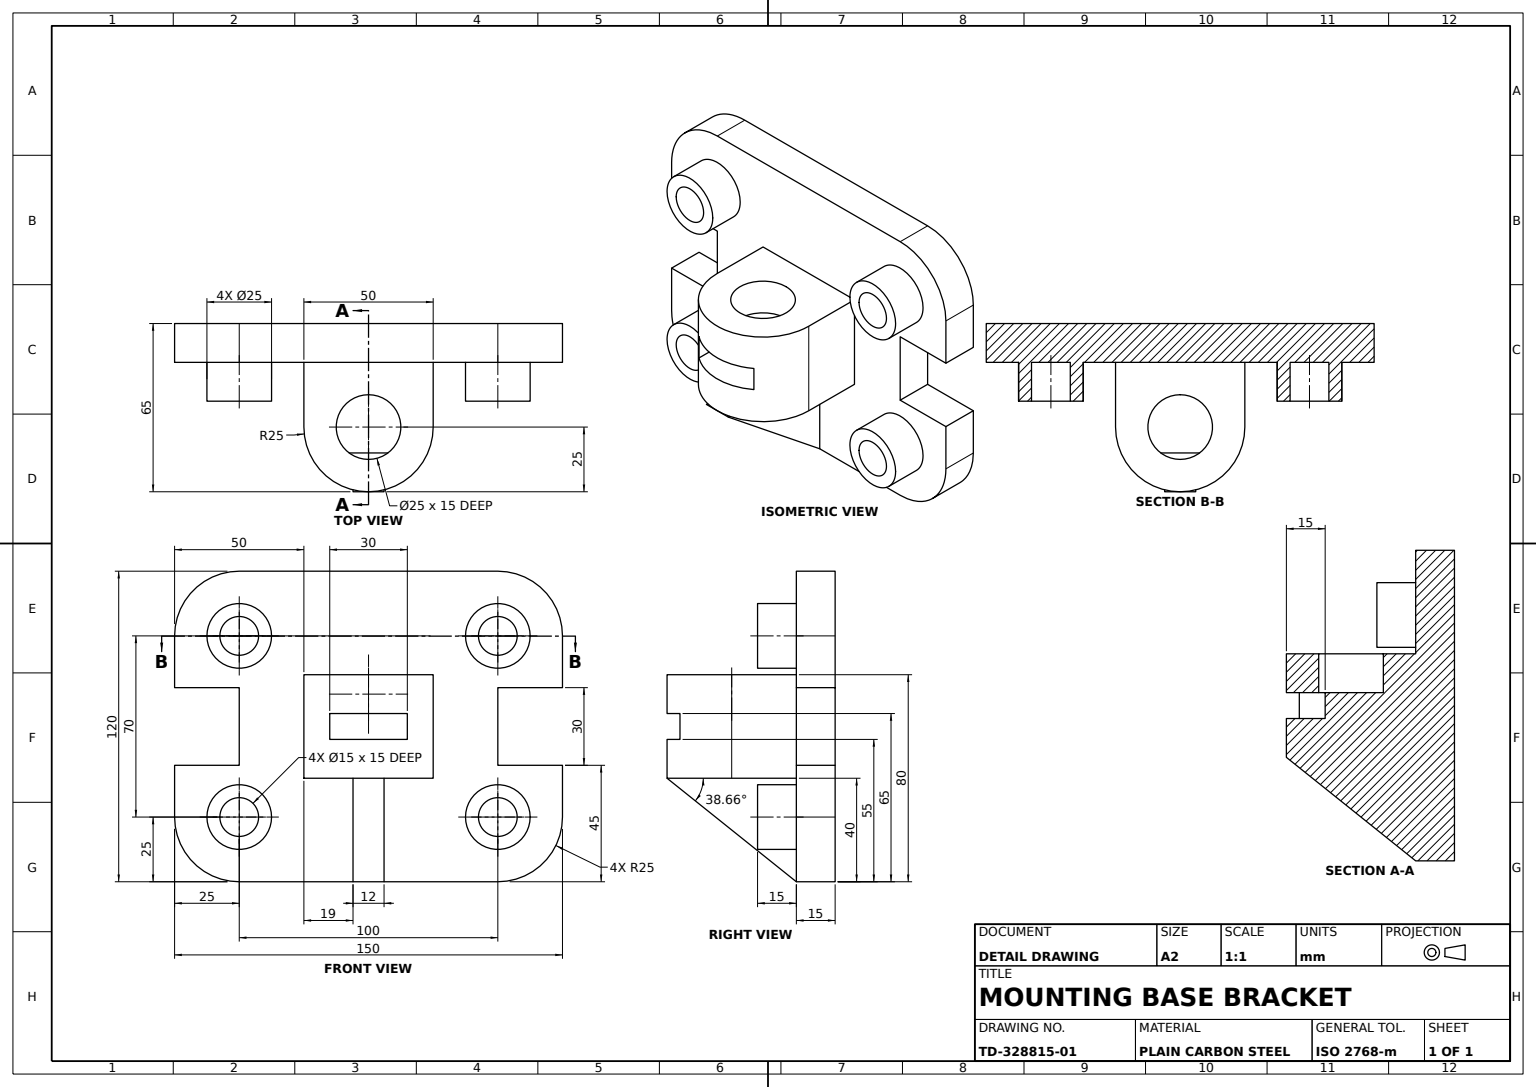
ISO-10303-21;
HEADER;
FILE_DESCRIPTION((''),'2;1');
FILE_NAME('','',(''),(''),'','','');
FILE_SCHEMA(('AUTOMOTIVE_DESIGN'));
ENDSEC;
DATA;
#1=APPLICATION_CONTEXT('');
#2=PRODUCT_CONTEXT('',#1,'mechanical');
#3=PRODUCT('','','',(#2));
#4=PRODUCT_DEFINITION_FORMATION('','',#3);
#5=PRODUCT_DEFINITION_CONTEXT('',#1,'design');
#6=PRODUCT_DEFINITION('','',#4,#5);
#7=PRODUCT_DEFINITION_SHAPE('','',#6);
#8=(LENGTH_UNIT()NAMED_UNIT(*)SI_UNIT(.MILLI.,.METRE.));
#9=(NAMED_UNIT(*)PLANE_ANGLE_UNIT()SI_UNIT($,.RADIAN.));
#10=(NAMED_UNIT(*)SI_UNIT($,.STERADIAN.)SOLID_ANGLE_UNIT());
#11=UNCERTAINTY_MEASURE_WITH_UNIT(LENGTH_MEASURE(1.E-05),#8,'distance_accuracy_value','');
#12=(GEOMETRIC_REPRESENTATION_CONTEXT(3)GLOBAL_UNCERTAINTY_ASSIGNED_CONTEXT((#11))GLOBAL_UNIT_ASSIGNED_CONTEXT((#8,#9,#10))REPRESENTATION_CONTEXT('',''));
#13=CARTESIAN_POINT('',(17.5,95.,30.));
#14=VERTEX_POINT('',#13);
#15=CARTESIAN_POINT('',(32.5,95.,30.));
#16=VERTEX_POINT('',#15);
#17=CARTESIAN_POINT('',(25.,95.,30.));
#18=DIRECTION('',(0.,0.,1.));
#19=DIRECTION('',(1.,0.,0.));
#20=AXIS2_PLACEMENT_3D('',#17,#18,#19);
#21=CIRCLE('',#20,7.5);
#22=EDGE_CURVE('',#14,#16,#21,.T.);
#23=ORIENTED_EDGE('',*,*,#22,.F.);
#24=EDGE_CURVE('',#16,#14,#21,.T.);
#25=ORIENTED_EDGE('',*,*,#24,.F.);
#26=EDGE_LOOP('',(#23,#25));
#27=FACE_BOUND('',#26,.T.);
#28=CARTESIAN_POINT('',(37.5,95.,30.));
#29=VERTEX_POINT('',#28);
#30=CARTESIAN_POINT('',(12.5,95.,30.));
#31=VERTEX_POINT('',#30);
#32=CIRCLE('',#20,12.5);
#33=EDGE_CURVE('',#29,#31,#32,.T.);
#34=ORIENTED_EDGE('',*,*,#33,.T.);
#35=EDGE_CURVE('',#31,#29,#32,.T.);
#36=ORIENTED_EDGE('',*,*,#35,.T.);
#37=EDGE_LOOP('',(#34,#36));
#38=FACE_OUTER_BOUND('',#37,.T.);
#39=PLANE('',#20);
#40=ADVANCED_FACE('',(#27,#38),#39,.T.);
#41=CARTESIAN_POINT('',(60.,65.,60.));
#42=VERTEX_POINT('',#41);
#43=CARTESIAN_POINT('',(90.,65.,60.));
#44=VERTEX_POINT('',#43);
#45=CARTESIAN_POINT('',(75.,65.,40.));
#46=DIRECTION('',(0.,1.,0.));
#47=AXIS2_PLACEMENT_3D('',#45,#46,#18);
#48=CIRCLE('',#47,25.);
#49=EDGE_CURVE('',#42,#44,#48,.T.);
#50=ORIENTED_EDGE('',*,*,#49,.F.);
#51=CARTESIAN_POINT('',(60.,65.,50.));
#52=VERTEX_POINT('',#51);
#53=VECTOR('',#18,1000.);
#54=LINE('',#51,#53);
#55=EDGE_CURVE('',#52,#42,#54,.T.);
#56=ORIENTED_EDGE('',*,*,#55,.F.);
#57=CARTESIAN_POINT('',(67.5,65.,50.));
#58=VERTEX_POINT('',#57);
#59=DIRECTION('',(-1.,0.,0.));
#60=VECTOR('',#59,1000.);
#61=LINE('',#51,#60);
#62=EDGE_CURVE('',#58,#52,#61,.T.);
#63=ORIENTED_EDGE('',*,*,#62,.F.);
#64=CARTESIAN_POINT('',(75.,65.,52.5));
#65=VERTEX_POINT('',#64);
#66=CIRCLE('',#47,12.5);
#67=EDGE_CURVE('',#58,#65,#66,.T.);
#68=ORIENTED_EDGE('',*,*,#67,.T.);
#69=CARTESIAN_POINT('',(82.5,65.,50.));
#70=VERTEX_POINT('',#69);
#71=EDGE_CURVE('',#65,#70,#66,.T.);
#72=ORIENTED_EDGE('',*,*,#71,.T.);
#73=CARTESIAN_POINT('',(90.,65.,50.));
#74=VERTEX_POINT('',#73);
#75=EDGE_CURVE('',#74,#70,#61,.T.);
#76=ORIENTED_EDGE('',*,*,#75,.F.);
#77=LINE('',#73,#53);
#78=EDGE_CURVE('',#74,#44,#77,.T.);
#79=ORIENTED_EDGE('',*,*,#78,.T.);
#80=EDGE_LOOP('',(#50,#56,#63,#68,#72,#76,#79));
#81=FACE_OUTER_BOUND('',#80,.T.);
#82=AXIS2_PLACEMENT_3D('',#51,#46,#18);
#83=PLANE('',#82);
#84=ADVANCED_FACE('',(#81),#83,.F.);
#85=CARTESIAN_POINT('',(25.,120.,15.));
#86=VERTEX_POINT('',#85);
#87=CARTESIAN_POINT('',(0.,95.,15.));
#88=VERTEX_POINT('',#87);
#89=CARTESIAN_POINT('',(25.,95.,15.));
#90=AXIS2_PLACEMENT_3D('',#89,#18,#19);
#91=CIRCLE('',#90,25.);
#92=EDGE_CURVE('',#86,#88,#91,.T.);
#93=ORIENTED_EDGE('',*,*,#92,.F.);
#94=CARTESIAN_POINT('',(25.,120.,0.));
#95=VERTEX_POINT('',#94);
#96=LINE('',#85,#53);
#97=EDGE_CURVE('',#95,#86,#96,.T.);
#98=ORIENTED_EDGE('',*,*,#97,.F.);
#99=CARTESIAN_POINT('',(0.,95.,0.));
#100=VERTEX_POINT('',#99);
#101=CARTESIAN_POINT('',(25.,95.,0.));
#102=DIRECTION('',(0.,0.,-1.));
#103=AXIS2_PLACEMENT_3D('',#101,#102,#19);
#104=CIRCLE('',#103,25.);
#105=EDGE_CURVE('',#100,#95,#104,.T.);
#106=ORIENTED_EDGE('',*,*,#105,.F.);
#107=VECTOR('',#102,1000.);
#108=LINE('',#87,#107);
#109=EDGE_CURVE('',#88,#100,#108,.T.);
#110=ORIENTED_EDGE('',*,*,#109,.F.);
#111=EDGE_LOOP('',(#93,#98,#106,#110));
#112=FACE_OUTER_BOUND('',#111,.T.);
#113=AXIS2_PLACEMENT_3D('',#89,#102,#59);
#114=CYLINDRICAL_SURFACE('',#113,25.);
#115=ADVANCED_FACE('',(#112),#114,.T.);
#116=CARTESIAN_POINT('',(81.,40.,65.));
#117=VERTEX_POINT('',#116);
#118=CARTESIAN_POINT('',(81.,0.,15.));
#119=VERTEX_POINT('',#118);
#120=DIRECTION('',(0.,-0.624695048,-0.780868809));
#121=VECTOR('',#120,1000.);
#122=LINE('',#118,#121);
#123=EDGE_CURVE('',#117,#119,#122,.T.);
#124=ORIENTED_EDGE('',*,*,#123,.T.);
#125=CARTESIAN_POINT('',(81.,40.,15.));
#126=VERTEX_POINT('',#125);
#127=VECTOR('',#46,1000.);
#128=LINE('',#125,#127);
#129=EDGE_CURVE('',#119,#126,#128,.T.);
#130=ORIENTED_EDGE('',*,*,#129,.T.);
#131=CARTESIAN_POINT('',(81.,40.,64.269322));
#132=VERTEX_POINT('',#131);
#133=LINE('',#116,#53);
#134=EDGE_CURVE('',#126,#132,#133,.T.);
#135=ORIENTED_EDGE('',*,*,#134,.T.);
#136=EDGE_CURVE('',#132,#117,#133,.T.);
#137=ORIENTED_EDGE('',*,*,#136,.T.);
#138=EDGE_LOOP('',(#124,#130,#135,#137));
#139=FACE_OUTER_BOUND('',#138,.T.);
#140=CARTESIAN_POINT('',(81.,0.,0.));
#141=AXIS2_PLACEMENT_3D('',#140,#19,#102);
#142=PLANE('',#141);
#143=ADVANCED_FACE('',(#139),#142,.T.);
#144=CARTESIAN_POINT('',(0.,25.,0.));
#145=VERTEX_POINT('',#144);
#146=CARTESIAN_POINT('',(0.,25.,15.));
#147=VERTEX_POINT('',#146);
#148=LINE('',#146,#53);
#149=EDGE_CURVE('',#145,#147,#148,.T.);
#150=ORIENTED_EDGE('',*,*,#149,.T.);
#151=CARTESIAN_POINT('',(0.,45.,15.));
#152=VERTEX_POINT('',#151);
#153=CARTESIAN_POINT('',(0.,120.,15.));
#154=DIRECTION('',(0.,-1.,0.));
#155=VECTOR('',#154,1000.);
#156=LINE('',#153,#155);
#157=EDGE_CURVE('',#152,#147,#156,.T.);
#158=ORIENTED_EDGE('',*,*,#157,.F.);
#159=CARTESIAN_POINT('',(0.,45.,0.));
#160=VERTEX_POINT('',#159);
#161=LINE('',#159,#53);
#162=EDGE_CURVE('',#160,#152,#161,.T.);
#163=ORIENTED_EDGE('',*,*,#162,.F.);
#164=CARTESIAN_POINT('',(0.,120.,0.));
#165=LINE('',#164,#155);
#166=EDGE_CURVE('',#160,#145,#165,.T.);
#167=ORIENTED_EDGE('',*,*,#166,.T.);
#168=EDGE_LOOP('',(#150,#158,#163,#167));
#169=FACE_OUTER_BOUND('',#168,.T.);
#170=AXIS2_PLACEMENT_3D('',#153,#19,#102);
#171=PLANE('',#170);
#172=ADVANCED_FACE('',(#169),#171,.F.);
#173=CARTESIAN_POINT('',(132.5,95.,30.));
#174=VERTEX_POINT('',#173);
#175=CARTESIAN_POINT('',(132.5,95.,15.));
#176=VERTEX_POINT('',#175);
#177=LINE('',#173,#107);
#178=EDGE_CURVE('',#174,#176,#177,.T.);
#179=ORIENTED_EDGE('',*,*,#178,.F.);
#180=CARTESIAN_POINT('',(117.5,95.,30.));
#181=VERTEX_POINT('',#180);
#182=CARTESIAN_POINT('',(125.,95.,30.));
#183=AXIS2_PLACEMENT_3D('',#182,#18,#19);
#184=CIRCLE('',#183,7.5);
#185=EDGE_CURVE('',#174,#181,#184,.T.);
#186=ORIENTED_EDGE('',*,*,#185,.T.);
#187=CARTESIAN_POINT('',(117.5,95.,15.));
#188=VERTEX_POINT('',#187);
#189=LINE('',#180,#107);
#190=EDGE_CURVE('',#181,#188,#189,.T.);
#191=ORIENTED_EDGE('',*,*,#190,.T.);
#192=CARTESIAN_POINT('',(125.,95.,15.));
#193=AXIS2_PLACEMENT_3D('',#192,#102,#19);
#194=CIRCLE('',#193,7.5);
#195=EDGE_CURVE('',#188,#176,#194,.T.);
#196=ORIENTED_EDGE('',*,*,#195,.T.);
#197=EDGE_LOOP('',(#179,#186,#191,#196));
#198=FACE_OUTER_BOUND('',#197,.T.);
#199=AXIS2_PLACEMENT_3D('',#182,#102,#59);
#200=CYLINDRICAL_SURFACE('',#199,7.5);
#201=ADVANCED_FACE('',(#198),#200,.F.);
#202=CARTESIAN_POINT('',(60.,55.,50.));
#203=VERTEX_POINT('',#202);
#204=LINE('',#51,#155);
#205=EDGE_CURVE('',#52,#203,#204,.T.);
#206=ORIENTED_EDGE('',*,*,#205,.F.);
#207=ORIENTED_EDGE('',*,*,#55,.T.);
#208=CARTESIAN_POINT('',(60.,55.,60.));
#209=VERTEX_POINT('',#208);
#210=CARTESIAN_POINT('',(60.,80.,60.));
#211=LINE('',#210,#127);
#212=EDGE_CURVE('',#209,#42,#211,.T.);
#213=ORIENTED_EDGE('',*,*,#212,.F.);
#214=LINE('',#202,#53);
#215=EDGE_CURVE('',#203,#209,#214,.T.);
#216=ORIENTED_EDGE('',*,*,#215,.F.);
#217=EDGE_LOOP('',(#206,#207,#213,#216));
#218=FACE_OUTER_BOUND('',#217,.T.);
#219=AXIS2_PLACEMENT_3D('',#51,#59,#18);
#220=PLANE('',#219);
#221=ADVANCED_FACE('',(#218),#220,.F.);
#222=ORIENTED_EDGE('',*,*,#109,.T.);
#223=CARTESIAN_POINT('',(0.,75.,0.));
#224=VERTEX_POINT('',#223);
#225=EDGE_CURVE('',#100,#224,#165,.T.);
#226=ORIENTED_EDGE('',*,*,#225,.T.);
#227=CARTESIAN_POINT('',(0.,75.,15.));
#228=VERTEX_POINT('',#227);
#229=LINE('',#223,#53);
#230=EDGE_CURVE('',#224,#228,#229,.T.);
#231=ORIENTED_EDGE('',*,*,#230,.T.);
#232=EDGE_CURVE('',#88,#228,#156,.T.);
#233=ORIENTED_EDGE('',*,*,#232,.F.);
#234=EDGE_LOOP('',(#222,#226,#231,#233));
#235=FACE_OUTER_BOUND('',#234,.T.);
#236=ADVANCED_FACE('',(#235),#171,.F.);
#237=CARTESIAN_POINT('',(125.,120.,15.));
#238=VERTEX_POINT('',#237);
#239=CARTESIAN_POINT('',(125.,120.,0.));
#240=VERTEX_POINT('',#239);
#241=LINE('',#237,#107);
#242=EDGE_CURVE('',#238,#240,#241,.T.);
#243=ORIENTED_EDGE('',*,*,#242,.T.);
#244=CARTESIAN_POINT('',(150.,120.,0.));
#245=LINE('',#244,#60);
#246=EDGE_CURVE('',#240,#95,#245,.T.);
#247=ORIENTED_EDGE('',*,*,#246,.T.);
#248=ORIENTED_EDGE('',*,*,#97,.T.);
#249=CARTESIAN_POINT('',(150.,120.,15.));
#250=LINE('',#249,#60);
#251=EDGE_CURVE('',#238,#86,#250,.T.);
#252=ORIENTED_EDGE('',*,*,#251,.F.);
#253=EDGE_LOOP('',(#243,#247,#248,#252));
#254=FACE_OUTER_BOUND('',#253,.T.);
#255=AXIS2_PLACEMENT_3D('',#249,#154,#102);
#256=PLANE('',#255);
#257=ADVANCED_FACE('',(#254),#256,.F.);
#258=CARTESIAN_POINT('',(25.,75.,15.));
#259=VERTEX_POINT('',#258);
#260=LINE('',#227,#60);
#261=EDGE_CURVE('',#259,#228,#260,.T.);
#262=ORIENTED_EDGE('',*,*,#261,.T.);
#263=ORIENTED_EDGE('',*,*,#230,.F.);
#264=CARTESIAN_POINT('',(25.,75.,0.));
#265=VERTEX_POINT('',#264);
#266=LINE('',#223,#60);
#267=EDGE_CURVE('',#265,#224,#266,.T.);
#268=ORIENTED_EDGE('',*,*,#267,.F.);
#269=LINE('',#264,#53);
#270=EDGE_CURVE('',#265,#259,#269,.T.);
#271=ORIENTED_EDGE('',*,*,#270,.T.);
#272=EDGE_LOOP('',(#262,#263,#268,#271));
#273=FACE_OUTER_BOUND('',#272,.T.);
#274=AXIS2_PLACEMENT_3D('',#223,#46,#18);
#275=PLANE('',#274);
#276=ADVANCED_FACE('',(#273),#275,.F.);
#277=CARTESIAN_POINT('',(100.,80.,15.));
#278=VERTEX_POINT('',#277);
#279=CARTESIAN_POINT('',(100.,40.,15.));
#280=VERTEX_POINT('',#279);
#281=LINE('',#277,#155);
#282=EDGE_CURVE('',#278,#280,#281,.T.);
#283=ORIENTED_EDGE('',*,*,#282,.F.);
#284=CARTESIAN_POINT('',(100.,80.,40.));
#285=VERTEX_POINT('',#284);
#286=LINE('',#284,#107);
#287=EDGE_CURVE('',#285,#278,#286,.T.);
#288=ORIENTED_EDGE('',*,*,#287,.F.);
#289=CARTESIAN_POINT('',(100.,40.,40.));
#290=VERTEX_POINT('',#289);
#291=LINE('',#284,#155);
#292=EDGE_CURVE('',#285,#290,#291,.T.);
#293=ORIENTED_EDGE('',*,*,#292,.T.);
#294=LINE('',#289,#107);
#295=EDGE_CURVE('',#290,#280,#294,.T.);
#296=ORIENTED_EDGE('',*,*,#295,.T.);
#297=EDGE_LOOP('',(#283,#288,#293,#296));
#298=FACE_OUTER_BOUND('',#297,.T.);
#299=AXIS2_PLACEMENT_3D('',#284,#59,#18);
#300=PLANE('',#299);
#301=ADVANCED_FACE('',(#298),#300,.F.);
#302=CARTESIAN_POINT('',(117.5,25.,15.));
#303=VERTEX_POINT('',#302);
#304=CARTESIAN_POINT('',(132.5,25.,15.));
#305=VERTEX_POINT('',#304);
#306=CARTESIAN_POINT('',(125.,25.,15.));
#307=AXIS2_PLACEMENT_3D('',#306,#102,#19);
#308=CIRCLE('',#307,7.5);
#309=EDGE_CURVE('',#303,#305,#308,.T.);
#310=ORIENTED_EDGE('',*,*,#309,.F.);
#311=EDGE_CURVE('',#305,#303,#308,.T.);
#312=ORIENTED_EDGE('',*,*,#311,.F.);
#313=EDGE_LOOP('',(#310,#312));
#314=FACE_OUTER_BOUND('',#313,.T.);
#315=CARTESIAN_POINT('',(0.,0.,15.));
#316=AXIS2_PLACEMENT_3D('',#315,#18,#19);
#317=PLANE('',#316);
#318=ADVANCED_FACE('',(#314),#317,.T.);
#319=CARTESIAN_POINT('',(125.,0.,0.));
#320=VERTEX_POINT('',#319);
#321=CARTESIAN_POINT('',(125.,0.,15.));
#322=VERTEX_POINT('',#321);
#323=LINE('',#321,#53);
#324=EDGE_CURVE('',#320,#322,#323,.T.);
#325=ORIENTED_EDGE('',*,*,#324,.F.);
#326=CARTESIAN_POINT('',(150.,25.,0.));
#327=VERTEX_POINT('',#326);
#328=CARTESIAN_POINT('',(125.,25.,0.));
#329=AXIS2_PLACEMENT_3D('',#328,#102,#19);
#330=CIRCLE('',#329,25.);
#331=EDGE_CURVE('',#327,#320,#330,.T.);
#332=ORIENTED_EDGE('',*,*,#331,.F.);
#333=CARTESIAN_POINT('',(150.,25.,15.));
#334=VERTEX_POINT('',#333);
#335=LINE('',#333,#107);
#336=EDGE_CURVE('',#334,#327,#335,.T.);
#337=ORIENTED_EDGE('',*,*,#336,.F.);
#338=AXIS2_PLACEMENT_3D('',#306,#18,#19);
#339=CIRCLE('',#338,25.);
#340=EDGE_CURVE('',#322,#334,#339,.T.);
#341=ORIENTED_EDGE('',*,*,#340,.F.);
#342=EDGE_LOOP('',(#325,#332,#337,#341));
#343=FACE_OUTER_BOUND('',#342,.T.);
#344=AXIS2_PLACEMENT_3D('',#306,#102,#59);
#345=CYLINDRICAL_SURFACE('',#344,25.);
#346=ADVANCED_FACE('',(#343),#345,.T.);
#347=CARTESIAN_POINT('',(75.,40.,65.));
#348=VERTEX_POINT('',#347);
#349=CARTESIAN_POINT('',(75.,40.,40.));
#350=AXIS2_PLACEMENT_3D('',#349,#46,#18);
#351=CIRCLE('',#350,25.);
#352=EDGE_CURVE('',#348,#132,#351,.T.);
#353=ORIENTED_EDGE('',*,*,#352,.F.);
#354=LINE('',#116,#60);
#355=EDGE_CURVE('',#117,#348,#354,.T.);
#356=ORIENTED_EDGE('',*,*,#355,.F.);
#357=ORIENTED_EDGE('',*,*,#136,.F.);
#358=EDGE_LOOP('',(#353,#356,#357));
#359=FACE_OUTER_BOUND('',#358,.T.);
#360=AXIS2_PLACEMENT_3D('',#116,#154,#102);
#361=PLANE('',#360);
#362=ADVANCED_FACE('',(#359),#361,.F.);
#363=CARTESIAN_POINT('',(90.,55.,50.));
#364=VERTEX_POINT('',#363);
#365=CARTESIAN_POINT('',(90.,55.,60.));
#366=VERTEX_POINT('',#365);
#367=LINE('',#363,#53);
#368=EDGE_CURVE('',#364,#366,#367,.T.);
#369=ORIENTED_EDGE('',*,*,#368,.F.);
#370=VECTOR('',#19,1000.);
#371=LINE('',#363,#370);
#372=EDGE_CURVE('',#203,#364,#371,.T.);
#373=ORIENTED_EDGE('',*,*,#372,.F.);
#374=ORIENTED_EDGE('',*,*,#215,.T.);
#375=CARTESIAN_POINT('',(75.,55.,40.));
#376=AXIS2_PLACEMENT_3D('',#375,#154,#102);
#377=CIRCLE('',#376,25.);
#378=EDGE_CURVE('',#366,#209,#377,.T.);
#379=ORIENTED_EDGE('',*,*,#378,.F.);
#380=EDGE_LOOP('',(#369,#373,#374,#379));
#381=FACE_OUTER_BOUND('',#380,.T.);
#382=AXIS2_PLACEMENT_3D('',#363,#154,#102);
#383=PLANE('',#382);
#384=ADVANCED_FACE('',(#381),#383,.F.);
#385=CARTESIAN_POINT('',(17.5,95.,15.));
#386=VERTEX_POINT('',#385);
#387=CARTESIAN_POINT('',(32.5,95.,15.));
#388=VERTEX_POINT('',#387);
#389=AXIS2_PLACEMENT_3D('',#89,#102,#19);
#390=CIRCLE('',#389,7.5);
#391=EDGE_CURVE('',#386,#388,#390,.T.);
#392=ORIENTED_EDGE('',*,*,#391,.T.);
#393=LINE('',#15,#107);
#394=EDGE_CURVE('',#16,#388,#393,.T.);
#395=ORIENTED_EDGE('',*,*,#394,.F.);
#396=ORIENTED_EDGE('',*,*,#24,.T.);
#397=LINE('',#13,#107);
#398=EDGE_CURVE('',#14,#386,#397,.T.);
#399=ORIENTED_EDGE('',*,*,#398,.T.);
#400=EDGE_LOOP('',(#392,#395,#396,#399));
#401=FACE_OUTER_BOUND('',#400,.T.);
#402=AXIS2_PLACEMENT_3D('',#17,#102,#59);
#403=CYLINDRICAL_SURFACE('',#402,7.5);
#404=ADVANCED_FACE('',(#401),#403,.F.);
#405=ORIENTED_EDGE('',*,*,#295,.F.);
#406=EDGE_CURVE('',#132,#290,#351,.T.);
#407=ORIENTED_EDGE('',*,*,#406,.F.);
#408=ORIENTED_EDGE('',*,*,#134,.F.);
#409=CARTESIAN_POINT('',(50.,40.,15.));
#410=LINE('',#409,#60);
#411=EDGE_CURVE('',#280,#126,#410,.T.);
#412=ORIENTED_EDGE('',*,*,#411,.F.);
#413=EDGE_LOOP('',(#405,#407,#408,#412));
#414=FACE_OUTER_BOUND('',#413,.T.);
#415=PLANE('',#350);
#416=ADVANCED_FACE('',(#414),#415,.F.);
#417=CARTESIAN_POINT('',(75.,80.,52.5));
#418=VERTEX_POINT('',#417);
#419=LINE('',#64,#127);
#420=EDGE_CURVE('',#65,#418,#419,.T.);
#421=ORIENTED_EDGE('',*,*,#420,.T.);
#422=CARTESIAN_POINT('',(75.,80.,27.5));
#423=VERTEX_POINT('',#422);
#424=CARTESIAN_POINT('',(75.,80.,40.));
#425=AXIS2_PLACEMENT_3D('',#424,#46,#18);
#426=CIRCLE('',#425,12.5);
#427=EDGE_CURVE('',#418,#423,#426,.T.);
#428=ORIENTED_EDGE('',*,*,#427,.T.);
#429=CARTESIAN_POINT('',(75.,65.,27.5));
#430=VERTEX_POINT('',#429);
#431=LINE('',#429,#127);
#432=EDGE_CURVE('',#430,#423,#431,.T.);
#433=ORIENTED_EDGE('',*,*,#432,.F.);
#434=EDGE_CURVE('',#70,#430,#66,.T.);
#435=ORIENTED_EDGE('',*,*,#434,.F.);
#436=ORIENTED_EDGE('',*,*,#71,.F.);
#437=EDGE_LOOP('',(#421,#428,#433,#435,#436));
#438=FACE_OUTER_BOUND('',#437,.T.);
#439=CYLINDRICAL_SURFACE('',#47,12.5);
#440=ADVANCED_FACE('',(#438),#439,.F.);
#441=CARTESIAN_POINT('',(125.,45.,0.));
#442=VERTEX_POINT('',#441);
#443=CARTESIAN_POINT('',(150.,45.,0.));
#444=VERTEX_POINT('',#443);
#445=LINE('',#441,#370);
#446=EDGE_CURVE('',#442,#444,#445,.T.);
#447=ORIENTED_EDGE('',*,*,#446,.F.);
#448=CARTESIAN_POINT('',(125.,45.,15.));
#449=VERTEX_POINT('',#448);
#450=LINE('',#441,#53);
#451=EDGE_CURVE('',#442,#449,#450,.T.);
#452=ORIENTED_EDGE('',*,*,#451,.T.);
#453=CARTESIAN_POINT('',(150.,45.,15.));
#454=VERTEX_POINT('',#453);
#455=LINE('',#448,#370);
#456=EDGE_CURVE('',#449,#454,#455,.T.);
#457=ORIENTED_EDGE('',*,*,#456,.T.);
#458=LINE('',#443,#53);
#459=EDGE_CURVE('',#444,#454,#458,.T.);
#460=ORIENTED_EDGE('',*,*,#459,.F.);
#461=EDGE_LOOP('',(#447,#452,#457,#460));
#462=FACE_OUTER_BOUND('',#461,.T.);
#463=AXIS2_PLACEMENT_3D('',#441,#154,#102);
#464=PLANE('',#463);
#465=ADVANCED_FACE('',(#462),#464,.F.);
#466=CARTESIAN_POINT('',(132.5,25.,30.));
#467=VERTEX_POINT('',#466);
#468=CARTESIAN_POINT('',(117.5,25.,30.));
#469=VERTEX_POINT('',#468);
#470=CARTESIAN_POINT('',(125.,25.,30.));
#471=AXIS2_PLACEMENT_3D('',#470,#18,#19);
#472=CIRCLE('',#471,7.5);
#473=EDGE_CURVE('',#467,#469,#472,.T.);
#474=ORIENTED_EDGE('',*,*,#473,.T.);
#475=LINE('',#468,#107);
#476=EDGE_CURVE('',#469,#303,#475,.T.);
#477=ORIENTED_EDGE('',*,*,#476,.T.);
#478=ORIENTED_EDGE('',*,*,#309,.T.);
#479=LINE('',#466,#107);
#480=EDGE_CURVE('',#467,#305,#479,.T.);
#481=ORIENTED_EDGE('',*,*,#480,.F.);
#482=EDGE_LOOP('',(#474,#477,#478,#481));
#483=FACE_OUTER_BOUND('',#482,.T.);
#484=AXIS2_PLACEMENT_3D('',#470,#102,#59);
#485=CYLINDRICAL_SURFACE('',#484,7.5);
#486=ADVANCED_FACE('',(#483),#485,.F.);
#487=ORIENTED_EDGE('',*,*,#67,.F.);
#488=EDGE_CURVE('',#430,#58,#66,.T.);
#489=ORIENTED_EDGE('',*,*,#488,.F.);
#490=ORIENTED_EDGE('',*,*,#432,.T.);
#491=EDGE_CURVE('',#423,#418,#426,.T.);
#492=ORIENTED_EDGE('',*,*,#491,.T.);
#493=ORIENTED_EDGE('',*,*,#420,.F.);
#494=EDGE_LOOP('',(#487,#489,#490,#492,#493));
#495=FACE_OUTER_BOUND('',#494,.T.);
#496=ADVANCED_FACE('',(#495),#439,.F.);
#497=ORIENTED_EDGE('',*,*,#242,.F.);
#498=CARTESIAN_POINT('',(150.,95.,15.));
#499=VERTEX_POINT('',#498);
#500=AXIS2_PLACEMENT_3D('',#192,#18,#19);
#501=CIRCLE('',#500,25.);
#502=EDGE_CURVE('',#499,#238,#501,.T.);
#503=ORIENTED_EDGE('',*,*,#502,.F.);
#504=CARTESIAN_POINT('',(150.,95.,0.));
#505=VERTEX_POINT('',#504);
#506=LINE('',#498,#53);
#507=EDGE_CURVE('',#505,#499,#506,.T.);
#508=ORIENTED_EDGE('',*,*,#507,.F.);
#509=CARTESIAN_POINT('',(125.,95.,0.));
#510=AXIS2_PLACEMENT_3D('',#509,#102,#19);
#511=CIRCLE('',#510,25.);
#512=EDGE_CURVE('',#240,#505,#511,.T.);
#513=ORIENTED_EDGE('',*,*,#512,.F.);
#514=EDGE_LOOP('',(#497,#503,#508,#513));
#515=FACE_OUTER_BOUND('',#514,.T.);
#516=AXIS2_PLACEMENT_3D('',#192,#102,#59);
#517=CYLINDRICAL_SURFACE('',#516,25.);
#518=ADVANCED_FACE('',(#515),#517,.T.);
#519=ORIENTED_EDGE('',*,*,#123,.F.);
#520=ORIENTED_EDGE('',*,*,#355,.T.);
#521=CARTESIAN_POINT('',(69.,40.,65.));
#522=VERTEX_POINT('',#521);
#523=EDGE_CURVE('',#348,#522,#354,.T.);
#524=ORIENTED_EDGE('',*,*,#523,.T.);
#525=CARTESIAN_POINT('',(69.,0.,15.));
#526=VERTEX_POINT('',#525);
#527=LINE('',#525,#121);
#528=EDGE_CURVE('',#522,#526,#527,.T.);
#529=ORIENTED_EDGE('',*,*,#528,.T.);
#530=LINE('',#118,#60);
#531=EDGE_CURVE('',#119,#526,#530,.T.);
#532=ORIENTED_EDGE('',*,*,#531,.F.);
#533=EDGE_LOOP('',(#519,#520,#524,#529,#532));
#534=FACE_OUTER_BOUND('',#533,.T.);
#535=DIRECTION('',(0.,0.780868809,-0.624695048));
#536=DIRECTION('',(0.,0.624695048,0.780868809));
#537=AXIS2_PLACEMENT_3D('',#118,#535,#536);
#538=PLANE('',#537);
#539=ADVANCED_FACE('',(#534),#538,.F.);
#540=CARTESIAN_POINT('',(69.,40.,64.269322));
#541=VERTEX_POINT('',#540);
#542=EDGE_CURVE('',#541,#348,#351,.T.);
#543=ORIENTED_EDGE('',*,*,#542,.T.);
#544=ORIENTED_EDGE('',*,*,#352,.T.);
#545=ORIENTED_EDGE('',*,*,#406,.T.);
#546=ORIENTED_EDGE('',*,*,#292,.F.);
#547=CARTESIAN_POINT('',(50.,80.,40.));
#548=VERTEX_POINT('',#547);
#549=CIRCLE('',#425,25.);
#550=EDGE_CURVE('',#548,#285,#549,.T.);
#551=ORIENTED_EDGE('',*,*,#550,.F.);
#552=CARTESIAN_POINT('',(50.,40.,40.));
#553=VERTEX_POINT('',#552);
#554=LINE('',#547,#155);
#555=EDGE_CURVE('',#548,#553,#554,.T.);
#556=ORIENTED_EDGE('',*,*,#555,.T.);
#557=EDGE_CURVE('',#553,#541,#351,.T.);
#558=ORIENTED_EDGE('',*,*,#557,.T.);
#559=EDGE_LOOP('',(#543,#544,#545,#546,#551,#556,#558));
#560=FACE_OUTER_BOUND('',#559,.T.);
#561=ORIENTED_EDGE('',*,*,#212,.T.);
#562=ORIENTED_EDGE('',*,*,#49,.T.);
#563=CARTESIAN_POINT('',(90.,80.,60.));
#564=LINE('',#563,#155);
#565=EDGE_CURVE('',#44,#366,#564,.T.);
#566=ORIENTED_EDGE('',*,*,#565,.T.);
#567=ORIENTED_EDGE('',*,*,#378,.T.);
#568=EDGE_LOOP('',(#561,#562,#566,#567));
#569=FACE_BOUND('',#568,.T.);
#570=AXIS2_PLACEMENT_3D('',#424,#154,#102);
#571=CYLINDRICAL_SURFACE('',#570,25.);
#572=ADVANCED_FACE('',(#560,#569),#571,.T.);
#573=CARTESIAN_POINT('',(112.5,25.,15.));
#574=VERTEX_POINT('',#573);
#575=CARTESIAN_POINT('',(137.5,25.,15.));
#576=VERTEX_POINT('',#575);
#577=CIRCLE('',#338,12.5);
#578=EDGE_CURVE('',#574,#576,#577,.T.);
#579=ORIENTED_EDGE('',*,*,#578,.T.);
#580=CARTESIAN_POINT('',(137.5,25.,30.));
#581=VERTEX_POINT('',#580);
#582=LINE('',#580,#107);
#583=EDGE_CURVE('',#581,#576,#582,.T.);
#584=ORIENTED_EDGE('',*,*,#583,.F.);
#585=CARTESIAN_POINT('',(112.5,25.,30.));
#586=VERTEX_POINT('',#585);
#587=CIRCLE('',#471,12.5);
#588=EDGE_CURVE('',#586,#581,#587,.T.);
#589=ORIENTED_EDGE('',*,*,#588,.F.);
#590=LINE('',#585,#107);
#591=EDGE_CURVE('',#586,#574,#590,.T.);
#592=ORIENTED_EDGE('',*,*,#591,.T.);
#593=EDGE_LOOP('',(#579,#584,#589,#592));
#594=FACE_OUTER_BOUND('',#593,.T.);
#595=CYLINDRICAL_SURFACE('',#484,12.5);
#596=ADVANCED_FACE('',(#594),#595,.T.);
#597=ORIENTED_EDGE('',*,*,#33,.F.);
#598=CARTESIAN_POINT('',(37.5,95.,15.));
#599=VERTEX_POINT('',#598);
#600=LINE('',#28,#107);
#601=EDGE_CURVE('',#29,#599,#600,.T.);
#602=ORIENTED_EDGE('',*,*,#601,.T.);
#603=CARTESIAN_POINT('',(12.5,95.,15.));
#604=VERTEX_POINT('',#603);
#605=CIRCLE('',#90,12.5);
#606=EDGE_CURVE('',#599,#604,#605,.T.);
#607=ORIENTED_EDGE('',*,*,#606,.T.);
#608=LINE('',#30,#107);
#609=EDGE_CURVE('',#31,#604,#608,.T.);
#610=ORIENTED_EDGE('',*,*,#609,.F.);
#611=EDGE_LOOP('',(#597,#602,#607,#610));
#612=FACE_OUTER_BOUND('',#611,.T.);
#613=CYLINDRICAL_SURFACE('',#402,12.5);
#614=ADVANCED_FACE('',(#612),#613,.T.);
#615=ORIENTED_EDGE('',*,*,#609,.T.);
#616=EDGE_CURVE('',#604,#599,#605,.T.);
#617=ORIENTED_EDGE('',*,*,#616,.T.);
#618=ORIENTED_EDGE('',*,*,#601,.F.);
#619=ORIENTED_EDGE('',*,*,#35,.F.);
#620=EDGE_LOOP('',(#615,#617,#618,#619));
#621=FACE_OUTER_BOUND('',#620,.T.);
#622=ADVANCED_FACE('',(#621),#613,.T.);
#623=CARTESIAN_POINT('',(112.5,95.,30.));
#624=VERTEX_POINT('',#623);
#625=CARTESIAN_POINT('',(112.5,95.,15.));
#626=VERTEX_POINT('',#625);
#627=LINE('',#623,#107);
#628=EDGE_CURVE('',#624,#626,#627,.T.);
#629=ORIENTED_EDGE('',*,*,#628,.T.);
#630=CARTESIAN_POINT('',(137.5,95.,15.));
#631=VERTEX_POINT('',#630);
#632=CIRCLE('',#500,12.5);
#633=EDGE_CURVE('',#626,#631,#632,.T.);
#634=ORIENTED_EDGE('',*,*,#633,.T.);
#635=CARTESIAN_POINT('',(137.5,95.,30.));
#636=VERTEX_POINT('',#635);
#637=LINE('',#635,#107);
#638=EDGE_CURVE('',#636,#631,#637,.T.);
#639=ORIENTED_EDGE('',*,*,#638,.F.);
#640=CIRCLE('',#183,12.5);
#641=EDGE_CURVE('',#624,#636,#640,.T.);
#642=ORIENTED_EDGE('',*,*,#641,.F.);
#643=EDGE_LOOP('',(#629,#634,#639,#642));
#644=FACE_OUTER_BOUND('',#643,.T.);
#645=CYLINDRICAL_SURFACE('',#199,12.5);
#646=ADVANCED_FACE('',(#644),#645,.T.);
#647=CARTESIAN_POINT('',(12.5,25.,30.));
#648=VERTEX_POINT('',#647);
#649=CARTESIAN_POINT('',(37.5,25.,30.));
#650=VERTEX_POINT('',#649);
#651=CARTESIAN_POINT('',(25.,25.,30.));
#652=AXIS2_PLACEMENT_3D('',#651,#18,#19);
#653=CIRCLE('',#652,12.5);
#654=EDGE_CURVE('',#648,#650,#653,.T.);
#655=ORIENTED_EDGE('',*,*,#654,.F.);
#656=CARTESIAN_POINT('',(12.5,25.,15.));
#657=VERTEX_POINT('',#656);
#658=LINE('',#647,#107);
#659=EDGE_CURVE('',#648,#657,#658,.T.);
#660=ORIENTED_EDGE('',*,*,#659,.T.);
#661=CARTESIAN_POINT('',(37.5,25.,15.));
#662=VERTEX_POINT('',#661);
#663=CARTESIAN_POINT('',(25.,25.,15.));
#664=AXIS2_PLACEMENT_3D('',#663,#18,#19);
#665=CIRCLE('',#664,12.5);
#666=EDGE_CURVE('',#657,#662,#665,.T.);
#667=ORIENTED_EDGE('',*,*,#666,.T.);
#668=LINE('',#649,#107);
#669=EDGE_CURVE('',#650,#662,#668,.T.);
#670=ORIENTED_EDGE('',*,*,#669,.F.);
#671=EDGE_LOOP('',(#655,#660,#667,#670));
#672=FACE_OUTER_BOUND('',#671,.T.);
#673=AXIS2_PLACEMENT_3D('',#651,#102,#59);
#674=CYLINDRICAL_SURFACE('',#673,12.5);
#675=ADVANCED_FACE('',(#672),#674,.T.);
#676=CARTESIAN_POINT('',(25.,45.,0.));
#677=VERTEX_POINT('',#676);
#678=LINE('',#264,#127);
#679=EDGE_CURVE('',#677,#265,#678,.T.);
#680=ORIENTED_EDGE('',*,*,#679,.F.);
#681=CARTESIAN_POINT('',(25.,45.,15.));
#682=VERTEX_POINT('',#681);
#683=LINE('',#676,#53);
#684=EDGE_CURVE('',#677,#682,#683,.T.);
#685=ORIENTED_EDGE('',*,*,#684,.T.);
#686=LINE('',#258,#127);
#687=EDGE_CURVE('',#682,#259,#686,.T.);
#688=ORIENTED_EDGE('',*,*,#687,.T.);
#689=ORIENTED_EDGE('',*,*,#270,.F.);
#690=EDGE_LOOP('',(#680,#685,#688,#689));
#691=FACE_OUTER_BOUND('',#690,.T.);
#692=AXIS2_PLACEMENT_3D('',#264,#19,#102);
#693=PLANE('',#692);
#694=ADVANCED_FACE('',(#691),#693,.F.);
#695=EDGE_CURVE('',#176,#188,#194,.T.);
#696=ORIENTED_EDGE('',*,*,#695,.T.);
#697=ORIENTED_EDGE('',*,*,#190,.F.);
#698=EDGE_CURVE('',#181,#174,#184,.T.);
#699=ORIENTED_EDGE('',*,*,#698,.T.);
#700=ORIENTED_EDGE('',*,*,#178,.T.);
#701=EDGE_LOOP('',(#696,#697,#699,#700));
#702=FACE_OUTER_BOUND('',#701,.T.);
#703=ADVANCED_FACE('',(#702),#200,.F.);
#704=CARTESIAN_POINT('',(32.5,25.,30.));
#705=VERTEX_POINT('',#704);
#706=CARTESIAN_POINT('',(17.5,25.,30.));
#707=VERTEX_POINT('',#706);
#708=CIRCLE('',#652,7.5);
#709=EDGE_CURVE('',#705,#707,#708,.T.);
#710=ORIENTED_EDGE('',*,*,#709,.F.);
#711=EDGE_CURVE('',#707,#705,#708,.T.);
#712=ORIENTED_EDGE('',*,*,#711,.F.);
#713=EDGE_LOOP('',(#710,#712));
#714=FACE_BOUND('',#713,.T.);
#715=ORIENTED_EDGE('',*,*,#654,.T.);
#716=EDGE_CURVE('',#650,#648,#653,.T.);
#717=ORIENTED_EDGE('',*,*,#716,.T.);
#718=EDGE_LOOP('',(#715,#717));
#719=FACE_OUTER_BOUND('',#718,.T.);
#720=PLANE('',#652);
#721=ADVANCED_FACE('',(#714,#719),#720,.T.);
#722=EDGE_CURVE('',#469,#467,#472,.T.);
#723=ORIENTED_EDGE('',*,*,#722,.T.);
#724=ORIENTED_EDGE('',*,*,#480,.T.);
#725=ORIENTED_EDGE('',*,*,#311,.T.);
#726=ORIENTED_EDGE('',*,*,#476,.F.);
#727=EDGE_LOOP('',(#723,#724,#725,#726));
#728=FACE_OUTER_BOUND('',#727,.T.);
#729=ADVANCED_FACE('',(#728),#485,.F.);
#730=ORIENTED_EDGE('',*,*,#666,.F.);
#731=EDGE_CURVE('',#662,#657,#665,.T.);
#732=ORIENTED_EDGE('',*,*,#731,.F.);
#733=EDGE_LOOP('',(#730,#732));
#734=FACE_BOUND('',#733,.T.);
#735=EDGE_CURVE('',#631,#626,#632,.T.);
#736=ORIENTED_EDGE('',*,*,#735,.F.);
#737=ORIENTED_EDGE('',*,*,#633,.F.);
#738=EDGE_LOOP('',(#736,#737));
#739=FACE_BOUND('',#738,.T.);
#740=EDGE_CURVE('',#576,#574,#577,.T.);
#741=ORIENTED_EDGE('',*,*,#740,.F.);
#742=ORIENTED_EDGE('',*,*,#578,.F.);
#743=EDGE_LOOP('',(#741,#742));
#744=FACE_BOUND('',#743,.T.);
#745=ORIENTED_EDGE('',*,*,#606,.F.);
#746=ORIENTED_EDGE('',*,*,#616,.F.);
#747=EDGE_LOOP('',(#745,#746));
#748=FACE_BOUND('',#747,.T.);
#749=ORIENTED_EDGE('',*,*,#340,.T.);
#750=CARTESIAN_POINT('',(150.,0.,15.));
#751=LINE('',#750,#127);
#752=EDGE_CURVE('',#334,#454,#751,.T.);
#753=ORIENTED_EDGE('',*,*,#752,.T.);
#754=ORIENTED_EDGE('',*,*,#456,.F.);
#755=CARTESIAN_POINT('',(125.,75.,15.));
#756=VERTEX_POINT('',#755);
#757=LINE('',#755,#155);
#758=EDGE_CURVE('',#756,#449,#757,.T.);
#759=ORIENTED_EDGE('',*,*,#758,.F.);
#760=CARTESIAN_POINT('',(150.,75.,15.));
#761=VERTEX_POINT('',#760);
#762=LINE('',#760,#60);
#763=EDGE_CURVE('',#761,#756,#762,.T.);
#764=ORIENTED_EDGE('',*,*,#763,.F.);
#765=EDGE_CURVE('',#761,#499,#751,.T.);
#766=ORIENTED_EDGE('',*,*,#765,.T.);
#767=ORIENTED_EDGE('',*,*,#502,.T.);
#768=ORIENTED_EDGE('',*,*,#251,.T.);
#769=ORIENTED_EDGE('',*,*,#92,.T.);
#770=ORIENTED_EDGE('',*,*,#232,.T.);
#771=ORIENTED_EDGE('',*,*,#261,.F.);
#772=ORIENTED_EDGE('',*,*,#687,.F.);
#773=LINE('',#681,#370);
#774=EDGE_CURVE('',#152,#682,#773,.T.);
#775=ORIENTED_EDGE('',*,*,#774,.F.);
#776=ORIENTED_EDGE('',*,*,#157,.T.);
#777=CARTESIAN_POINT('',(25.,0.,15.));
#778=VERTEX_POINT('',#777);
#779=CIRCLE('',#664,25.);
#780=EDGE_CURVE('',#147,#778,#779,.T.);
#781=ORIENTED_EDGE('',*,*,#780,.T.);
#782=LINE('',#315,#370);
#783=EDGE_CURVE('',#778,#526,#782,.T.);
#784=ORIENTED_EDGE('',*,*,#783,.T.);
#785=CARTESIAN_POINT('',(69.,40.,15.));
#786=VERTEX_POINT('',#785);
#787=LINE('',#785,#127);
#788=EDGE_CURVE('',#526,#786,#787,.T.);
#789=ORIENTED_EDGE('',*,*,#788,.T.);
#790=VERTEX_POINT('',#409);
#791=EDGE_CURVE('',#786,#790,#410,.T.);
#792=ORIENTED_EDGE('',*,*,#791,.T.);
#793=CARTESIAN_POINT('',(50.,80.,15.));
#794=VERTEX_POINT('',#793);
#795=LINE('',#793,#155);
#796=EDGE_CURVE('',#794,#790,#795,.T.);
#797=ORIENTED_EDGE('',*,*,#796,.F.);
#798=LINE('',#793,#60);
#799=EDGE_CURVE('',#278,#794,#798,.T.);
#800=ORIENTED_EDGE('',*,*,#799,.F.);
#801=ORIENTED_EDGE('',*,*,#282,.T.);
#802=ORIENTED_EDGE('',*,*,#411,.T.);
#803=ORIENTED_EDGE('',*,*,#129,.F.);
#804=EDGE_CURVE('',#119,#322,#782,.T.);
#805=ORIENTED_EDGE('',*,*,#804,.T.);
#806=EDGE_LOOP('',(#749,#753,#754,#759,#764,#766,#767,#768,#769,#770,#771,#772,#775,#776,#781,#784,#789,#792,#797,#800,#801,#802,#803,#805));
#807=FACE_OUTER_BOUND('',#806,.T.);
#808=ADVANCED_FACE('',(#734,#739,#744,#748,#807),#317,.T.);
#809=ORIENTED_EDGE('',*,*,#695,.F.);
#810=ORIENTED_EDGE('',*,*,#195,.F.);
#811=EDGE_LOOP('',(#809,#810));
#812=FACE_OUTER_BOUND('',#811,.T.);
#813=ADVANCED_FACE('',(#812),#317,.T.);
#814=ORIENTED_EDGE('',*,*,#398,.F.);
#815=ORIENTED_EDGE('',*,*,#22,.T.);
#816=ORIENTED_EDGE('',*,*,#394,.T.);
#817=EDGE_CURVE('',#388,#386,#390,.T.);
#818=ORIENTED_EDGE('',*,*,#817,.T.);
#819=EDGE_LOOP('',(#814,#815,#816,#818));
#820=FACE_OUTER_BOUND('',#819,.T.);
#821=ADVANCED_FACE('',(#820),#403,.F.);
#822=ORIENTED_EDGE('',*,*,#166,.F.);
#823=LINE('',#676,#370);
#824=EDGE_CURVE('',#160,#677,#823,.T.);
#825=ORIENTED_EDGE('',*,*,#824,.T.);
#826=ORIENTED_EDGE('',*,*,#679,.T.);
#827=ORIENTED_EDGE('',*,*,#267,.T.);
#828=ORIENTED_EDGE('',*,*,#225,.F.);
#829=ORIENTED_EDGE('',*,*,#105,.T.);
#830=ORIENTED_EDGE('',*,*,#246,.F.);
#831=ORIENTED_EDGE('',*,*,#512,.T.);
#832=CARTESIAN_POINT('',(150.,75.,0.));
#833=VERTEX_POINT('',#832);
#834=CARTESIAN_POINT('',(150.,0.,0.));
#835=LINE('',#834,#127);
#836=EDGE_CURVE('',#833,#505,#835,.T.);
#837=ORIENTED_EDGE('',*,*,#836,.F.);
#838=CARTESIAN_POINT('',(125.,75.,0.));
#839=VERTEX_POINT('',#838);
#840=LINE('',#832,#60);
#841=EDGE_CURVE('',#833,#839,#840,.T.);
#842=ORIENTED_EDGE('',*,*,#841,.T.);
#843=LINE('',#838,#155);
#844=EDGE_CURVE('',#839,#442,#843,.T.);
#845=ORIENTED_EDGE('',*,*,#844,.T.);
#846=ORIENTED_EDGE('',*,*,#446,.T.);
#847=EDGE_CURVE('',#327,#444,#835,.T.);
#848=ORIENTED_EDGE('',*,*,#847,.F.);
#849=ORIENTED_EDGE('',*,*,#331,.T.);
#850=CARTESIAN_POINT('',(25.,0.,0.));
#851=VERTEX_POINT('',#850);
#852=CARTESIAN_POINT('',(0.,0.,0.));
#853=LINE('',#852,#370);
#854=EDGE_CURVE('',#851,#320,#853,.T.);
#855=ORIENTED_EDGE('',*,*,#854,.F.);
#856=CARTESIAN_POINT('',(25.,25.,0.));
#857=AXIS2_PLACEMENT_3D('',#856,#102,#19);
#858=CIRCLE('',#857,25.);
#859=EDGE_CURVE('',#851,#145,#858,.T.);
#860=ORIENTED_EDGE('',*,*,#859,.T.);
#861=EDGE_LOOP('',(#822,#825,#826,#827,#828,#829,#830,#831,#837,#842,#845,#846,#848,#849,#855,#860));
#862=FACE_OUTER_BOUND('',#861,.T.);
#863=AXIS2_PLACEMENT_3D('',#852,#18,#19);
#864=PLANE('',#863);
#865=ADVANCED_FACE('',(#862),#864,.F.);
#866=EDGE_CURVE('',#636,#624,#640,.T.);
#867=ORIENTED_EDGE('',*,*,#866,.T.);
#868=ORIENTED_EDGE('',*,*,#641,.T.);
#869=EDGE_LOOP('',(#867,#868));
#870=FACE_OUTER_BOUND('',#869,.T.);
#871=ORIENTED_EDGE('',*,*,#185,.F.);
#872=ORIENTED_EDGE('',*,*,#698,.F.);
#873=EDGE_LOOP('',(#871,#872));
#874=FACE_BOUND('',#873,.T.);
#875=PLANE('',#183);
#876=ADVANCED_FACE('',(#870,#874),#875,.T.);
#877=ORIENTED_EDGE('',*,*,#488,.T.);
#878=EDGE_CURVE('',#70,#58,#61,.T.);
#879=ORIENTED_EDGE('',*,*,#878,.F.);
#880=ORIENTED_EDGE('',*,*,#434,.T.);
#881=EDGE_LOOP('',(#877,#879,#880));
#882=FACE_OUTER_BOUND('',#881,.T.);
#883=PLANE('',#47);
#884=ADVANCED_FACE('',(#882),#883,.T.);
#885=ORIENTED_EDGE('',*,*,#752,.F.);
#886=ORIENTED_EDGE('',*,*,#336,.T.);
#887=ORIENTED_EDGE('',*,*,#847,.T.);
#888=ORIENTED_EDGE('',*,*,#459,.T.);
#889=EDGE_LOOP('',(#885,#886,#887,#888));
#890=FACE_OUTER_BOUND('',#889,.T.);
#891=AXIS2_PLACEMENT_3D('',#750,#59,#18);
#892=PLANE('',#891);
#893=ADVANCED_FACE('',(#890),#892,.F.);
#894=ORIENTED_EDGE('',*,*,#324,.T.);
#895=ORIENTED_EDGE('',*,*,#804,.F.);
#896=ORIENTED_EDGE('',*,*,#531,.T.);
#897=ORIENTED_EDGE('',*,*,#783,.F.);
#898=LINE('',#777,#107);
#899=EDGE_CURVE('',#778,#851,#898,.T.);
#900=ORIENTED_EDGE('',*,*,#899,.T.);
#901=ORIENTED_EDGE('',*,*,#854,.T.);
#902=EDGE_LOOP('',(#894,#895,#896,#897,#900,#901));
#903=FACE_OUTER_BOUND('',#902,.T.);
#904=AXIS2_PLACEMENT_3D('',#315,#46,#18);
#905=PLANE('',#904);
#906=ADVANCED_FACE('',(#903),#905,.F.);
#907=ORIENTED_EDGE('',*,*,#287,.T.);
#908=ORIENTED_EDGE('',*,*,#799,.T.);
#909=LINE('',#547,#53);
#910=EDGE_CURVE('',#794,#548,#909,.T.);
#911=ORIENTED_EDGE('',*,*,#910,.T.);
#912=ORIENTED_EDGE('',*,*,#550,.T.);
#913=EDGE_LOOP('',(#907,#908,#911,#912));
#914=FACE_OUTER_BOUND('',#913,.T.);
#915=ORIENTED_EDGE('',*,*,#427,.F.);
#916=ORIENTED_EDGE('',*,*,#491,.F.);
#917=EDGE_LOOP('',(#915,#916));
#918=FACE_BOUND('',#917,.T.);
#919=PLANE('',#425);
#920=ADVANCED_FACE('',(#914,#918),#919,.T.);
#921=ORIENTED_EDGE('',*,*,#788,.F.);
#922=ORIENTED_EDGE('',*,*,#528,.F.);
#923=LINE('',#521,#53);
#924=EDGE_CURVE('',#541,#522,#923,.T.);
#925=ORIENTED_EDGE('',*,*,#924,.F.);
#926=EDGE_CURVE('',#786,#541,#923,.T.);
#927=ORIENTED_EDGE('',*,*,#926,.F.);
#928=EDGE_LOOP('',(#921,#922,#925,#927));
#929=FACE_OUTER_BOUND('',#928,.T.);
#930=CARTESIAN_POINT('',(69.,0.,0.));
#931=AXIS2_PLACEMENT_3D('',#930,#19,#102);
#932=PLANE('',#931);
#933=ADVANCED_FACE('',(#929),#932,.F.);
#934=ORIENTED_EDGE('',*,*,#774,.T.);
#935=ORIENTED_EDGE('',*,*,#684,.F.);
#936=ORIENTED_EDGE('',*,*,#824,.F.);
#937=ORIENTED_EDGE('',*,*,#162,.T.);
#938=EDGE_LOOP('',(#934,#935,#936,#937));
#939=FACE_OUTER_BOUND('',#938,.T.);
#940=AXIS2_PLACEMENT_3D('',#676,#154,#102);
#941=PLANE('',#940);
#942=ADVANCED_FACE('',(#939),#941,.F.);
#943=ORIENTED_EDGE('',*,*,#555,.F.);
#944=ORIENTED_EDGE('',*,*,#910,.F.);
#945=ORIENTED_EDGE('',*,*,#796,.T.);
#946=LINE('',#552,#53);
#947=EDGE_CURVE('',#790,#553,#946,.T.);
#948=ORIENTED_EDGE('',*,*,#947,.T.);
#949=EDGE_LOOP('',(#943,#944,#945,#948));
#950=FACE_OUTER_BOUND('',#949,.T.);
#951=AXIS2_PLACEMENT_3D('',#547,#19,#102);
#952=PLANE('',#951);
#953=ADVANCED_FACE('',(#950),#952,.F.);
#954=LINE('',#832,#53);
#955=EDGE_CURVE('',#833,#761,#954,.T.);
#956=ORIENTED_EDGE('',*,*,#955,.F.);
#957=ORIENTED_EDGE('',*,*,#836,.T.);
#958=ORIENTED_EDGE('',*,*,#507,.T.);
#959=ORIENTED_EDGE('',*,*,#765,.F.);
#960=EDGE_LOOP('',(#956,#957,#958,#959));
#961=FACE_OUTER_BOUND('',#960,.T.);
#962=ADVANCED_FACE('',(#961),#892,.F.);
#963=ORIENTED_EDGE('',*,*,#451,.F.);
#964=ORIENTED_EDGE('',*,*,#844,.F.);
#965=LINE('',#838,#53);
#966=EDGE_CURVE('',#839,#756,#965,.T.);
#967=ORIENTED_EDGE('',*,*,#966,.T.);
#968=ORIENTED_EDGE('',*,*,#758,.T.);
#969=EDGE_LOOP('',(#963,#964,#967,#968));
#970=FACE_OUTER_BOUND('',#969,.T.);
#971=AXIS2_PLACEMENT_3D('',#838,#59,#18);
#972=PLANE('',#971);
#973=ADVANCED_FACE('',(#970),#972,.F.);
#974=CARTESIAN_POINT('',(32.5,25.,15.));
#975=VERTEX_POINT('',#974);
#976=LINE('',#704,#107);
#977=EDGE_CURVE('',#705,#975,#976,.T.);
#978=ORIENTED_EDGE('',*,*,#977,.F.);
#979=ORIENTED_EDGE('',*,*,#709,.T.);
#980=CARTESIAN_POINT('',(17.5,25.,15.));
#981=VERTEX_POINT('',#980);
#982=LINE('',#706,#107);
#983=EDGE_CURVE('',#707,#981,#982,.T.);
#984=ORIENTED_EDGE('',*,*,#983,.T.);
#985=AXIS2_PLACEMENT_3D('',#663,#102,#19);
#986=CIRCLE('',#985,7.5);
#987=EDGE_CURVE('',#981,#975,#986,.T.);
#988=ORIENTED_EDGE('',*,*,#987,.T.);
#989=EDGE_LOOP('',(#978,#979,#984,#988));
#990=FACE_OUTER_BOUND('',#989,.T.);
#991=CYLINDRICAL_SURFACE('',#673,7.5);
#992=ADVANCED_FACE('',(#990),#991,.F.);
#993=ORIENTED_EDGE('',*,*,#924,.T.);
#994=ORIENTED_EDGE('',*,*,#523,.F.);
#995=ORIENTED_EDGE('',*,*,#542,.F.);
#996=EDGE_LOOP('',(#993,#994,#995));
#997=FACE_OUTER_BOUND('',#996,.T.);
#998=ADVANCED_FACE('',(#997),#361,.F.);
#999=ORIENTED_EDGE('',*,*,#711,.T.);
#1000=ORIENTED_EDGE('',*,*,#977,.T.);
#1001=EDGE_CURVE('',#975,#981,#986,.T.);
#1002=ORIENTED_EDGE('',*,*,#1001,.T.);
#1003=ORIENTED_EDGE('',*,*,#983,.F.);
#1004=EDGE_LOOP('',(#999,#1000,#1002,#1003));
#1005=FACE_OUTER_BOUND('',#1004,.T.);
#1006=ADVANCED_FACE('',(#1005),#991,.F.);
#1007=ORIENTED_EDGE('',*,*,#583,.T.);
#1008=ORIENTED_EDGE('',*,*,#740,.T.);
#1009=ORIENTED_EDGE('',*,*,#591,.F.);
#1010=EDGE_CURVE('',#581,#586,#587,.T.);
#1011=ORIENTED_EDGE('',*,*,#1010,.F.);
#1012=EDGE_LOOP('',(#1007,#1008,#1009,#1011));
#1013=FACE_OUTER_BOUND('',#1012,.T.);
#1014=ADVANCED_FACE('',(#1013),#595,.T.);
#1015=ORIENTED_EDGE('',*,*,#75,.T.);
#1016=ORIENTED_EDGE('',*,*,#878,.T.);
#1017=ORIENTED_EDGE('',*,*,#62,.T.);
#1018=ORIENTED_EDGE('',*,*,#205,.T.);
#1019=ORIENTED_EDGE('',*,*,#372,.T.);
#1020=LINE('',#73,#127);
#1021=EDGE_CURVE('',#364,#74,#1020,.T.);
#1022=ORIENTED_EDGE('',*,*,#1021,.T.);
#1023=EDGE_LOOP('',(#1015,#1016,#1017,#1018,#1019,#1022));
#1024=FACE_OUTER_BOUND('',#1023,.T.);
#1025=CARTESIAN_POINT('',(0.,0.,50.));
#1026=AXIS2_PLACEMENT_3D('',#1025,#102,#59);
#1027=PLANE('',#1026);
#1028=ADVANCED_FACE('',(#1024),#1027,.F.);
#1029=ORIENTED_EDGE('',*,*,#473,.F.);
#1030=ORIENTED_EDGE('',*,*,#722,.F.);
#1031=EDGE_LOOP('',(#1029,#1030));
#1032=FACE_BOUND('',#1031,.T.);
#1033=ORIENTED_EDGE('',*,*,#588,.T.);
#1034=ORIENTED_EDGE('',*,*,#1010,.T.);
#1035=EDGE_LOOP('',(#1033,#1034));
#1036=FACE_OUTER_BOUND('',#1035,.T.);
#1037=PLANE('',#471);
#1038=ADVANCED_FACE('',(#1032,#1036),#1037,.T.);
#1039=ORIENTED_EDGE('',*,*,#780,.F.);
#1040=ORIENTED_EDGE('',*,*,#149,.F.);
#1041=ORIENTED_EDGE('',*,*,#859,.F.);
#1042=ORIENTED_EDGE('',*,*,#899,.F.);
#1043=EDGE_LOOP('',(#1039,#1040,#1041,#1042));
#1044=FACE_OUTER_BOUND('',#1043,.T.);
#1045=AXIS2_PLACEMENT_3D('',#663,#102,#59);
#1046=CYLINDRICAL_SURFACE('',#1045,25.);
#1047=ADVANCED_FACE('',(#1044),#1046,.T.);
#1048=ORIENTED_EDGE('',*,*,#866,.F.);
#1049=ORIENTED_EDGE('',*,*,#638,.T.);
#1050=ORIENTED_EDGE('',*,*,#735,.T.);
#1051=ORIENTED_EDGE('',*,*,#628,.F.);
#1052=EDGE_LOOP('',(#1048,#1049,#1050,#1051));
#1053=FACE_OUTER_BOUND('',#1052,.T.);
#1054=ADVANCED_FACE('',(#1053),#645,.T.);
#1055=ORIENTED_EDGE('',*,*,#817,.F.);
#1056=ORIENTED_EDGE('',*,*,#391,.F.);
#1057=EDGE_LOOP('',(#1055,#1056));
#1058=FACE_OUTER_BOUND('',#1057,.T.);
#1059=ADVANCED_FACE('',(#1058),#317,.T.);
#1060=ORIENTED_EDGE('',*,*,#791,.F.);
#1061=ORIENTED_EDGE('',*,*,#926,.T.);
#1062=ORIENTED_EDGE('',*,*,#557,.F.);
#1063=ORIENTED_EDGE('',*,*,#947,.F.);
#1064=EDGE_LOOP('',(#1060,#1061,#1062,#1063));
#1065=FACE_OUTER_BOUND('',#1064,.T.);
#1066=ADVANCED_FACE('',(#1065),#415,.F.);
#1067=ORIENTED_EDGE('',*,*,#763,.T.);
#1068=ORIENTED_EDGE('',*,*,#966,.F.);
#1069=ORIENTED_EDGE('',*,*,#841,.F.);
#1070=ORIENTED_EDGE('',*,*,#955,.T.);
#1071=EDGE_LOOP('',(#1067,#1068,#1069,#1070));
#1072=FACE_OUTER_BOUND('',#1071,.T.);
#1073=AXIS2_PLACEMENT_3D('',#832,#46,#18);
#1074=PLANE('',#1073);
#1075=ADVANCED_FACE('',(#1072),#1074,.F.);
#1076=ORIENTED_EDGE('',*,*,#659,.F.);
#1077=ORIENTED_EDGE('',*,*,#716,.F.);
#1078=ORIENTED_EDGE('',*,*,#669,.T.);
#1079=ORIENTED_EDGE('',*,*,#731,.T.);
#1080=EDGE_LOOP('',(#1076,#1077,#1078,#1079));
#1081=FACE_OUTER_BOUND('',#1080,.T.);
#1082=ADVANCED_FACE('',(#1081),#674,.T.);
#1083=ORIENTED_EDGE('',*,*,#78,.F.);
#1084=ORIENTED_EDGE('',*,*,#1021,.F.);
#1085=ORIENTED_EDGE('',*,*,#368,.T.);
#1086=ORIENTED_EDGE('',*,*,#565,.F.);
#1087=EDGE_LOOP('',(#1083,#1084,#1085,#1086));
#1088=FACE_OUTER_BOUND('',#1087,.T.);
#1089=AXIS2_PLACEMENT_3D('',#73,#19,#102);
#1090=PLANE('',#1089);
#1091=ADVANCED_FACE('',(#1088),#1090,.F.);
#1092=ORIENTED_EDGE('',*,*,#987,.F.);
#1093=ORIENTED_EDGE('',*,*,#1001,.F.);
#1094=EDGE_LOOP('',(#1092,#1093));
#1095=FACE_OUTER_BOUND('',#1094,.T.);
#1096=ADVANCED_FACE('',(#1095),#317,.T.);
#1097=CLOSED_SHELL('',(#40,#84,#115,#143,#172,#201,#221,#236,#257,#276,#301,#318,#346,#362,#384,#404,#416,#440,#465,#486,#496,#518,#539,#572,#596,#614,#622,#646,#675,#694,#703,#721,#729,#808,#813,#821,#865,#876,#884,#893,#906,#920,#933,#942,#953,#962,#973,#992,#998,#1006,#1014,#1028,#1038,#1047,#1054,#1059,#1066,#1075,#1082,#1091,#1096));
#1098=MANIFOLD_SOLID_BREP('',#1097);
#1099=ADVANCED_BREP_SHAPE_REPRESENTATION('',(#1098),#12);
#1100=SHAPE_DEFINITION_REPRESENTATION(#7,#1099);
ENDSEC;
END-ISO-10303-21;
